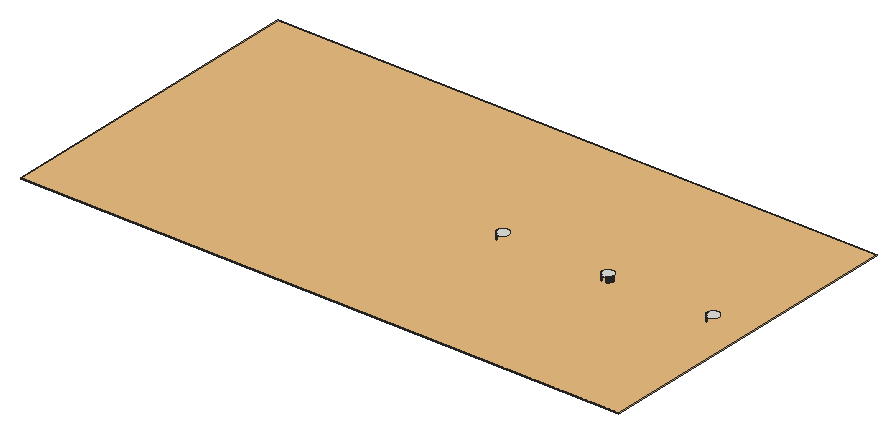
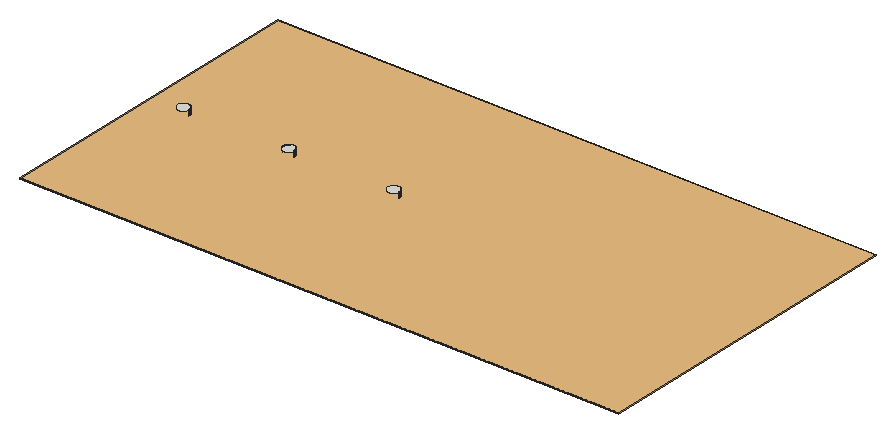
# SketchUp Ruby script. Lengths in inches.
U = 1.inch
M = Sketchup.active_model
def pt(a) = Geom::Point3d.new(a.map { |v| v * U })
def face(e, loops, mat)
  f = e.add_face(loops[0].map { |a| pt(a) })
  loops[1..].each { |l| e.add_face(l.map { |a| pt(a) }).erase! }
  f.material = f.back_material = mat if mat
  f
end
# faces: each face lists its corners as indices into pts; further lists are holes
def faces(e, pts, list, mat = nil) = list.each { |f| face(e, (f[0].is_a?(Array) ? f : [f]).map { |l| l.map { |i| pts[i] } }, mat) }
# xy, xz, yz: faces in a plane at the given z, y or x. An outline is a flat list of corners, or four numbers for a rectangle; further outlines are holes
def ring(l) = l.size == 4 ? [[l[0], l[1]], [l[2], l[1]], [l[2], l[3]], [l[0], l[3]]] : l.each_slice(2).to_a
def flat(e, list, mat, &to3) = list.each { |f| face(e, (f[0].is_a?(Array) ? f : [f]).map { |l| ring(l).map { |u, v| to3.(u, v) } }, mat) }
def xy(e, z, list, mat = nil) = flat(e, list, mat) { |x, y| [x, y, z] }
def xz(e, y, list, mat = nil) = flat(e, list, mat) { |x, z| [x, y, z] }
def yz(e, x, list, mat = nil) = flat(e, list, mat) { |y, z| [x, y, z] }
def lines(e, pts, list) = list.each { |a, b| e.add_line(pt(pts[a]), pt(pts[b])) }
# prism: a flat outline (further loops are holes) pulled along v
def prism(e, loops, v, mat = nil)
  f = face(e, loops, mat); d = Geom::Vector3d.new(v.map { |x| x * U })
  f.pushpull(f.normal.samedirection?(d) ? d.length : -d.length)
end
def box(e, o, s, mat = nil) = prism(e, [[o, [o[0] + s[0], o[1], o[2]], [o[0] + s[0], o[1] + s[1], o[2]], [o[0], o[1] + s[1], o[2]]]], [0, 0, s[2]], mat)
def at(x, y, z, deg = 0) = Geom::Transformation.translation(pt([x, y, z])) * Geom::Transformation.rotation(ORIGIN, Z_AXIS, deg.degrees)
def axes(o, x, y, z) = Geom::Transformation.new([*x, 0, *y, 0, *z, 0, *pt(o).to_a, 1])
def part(name) = M.definitions.add(name)
# library, detail: a bought-in or finely detailed component or shape, given as its bounding box
def library(name, o, s) = part(name).tap { |d| box(d.entities, o, s) }
def detail(e, o, s) = box(e.add_group.entities, o, s)
def put(e, d, t, mat = nil) = e.add_instance(d, t).tap { |i| i.material = mat if mat }
def group(e, t, mat = nil) = e.add_group.tap { |g| g.transformation = t; g.material = mat if mat }.entities
root = M.entities
M.materials.add("False Ceiling light").color = [253, 223, 143]
c1 = library("Group\#25",[0,0,-0.5],[312,168,0.5])
xy(root,234,[[214.28,251,214.2,251.01,214.12,251.01,213.96,251.03,213.89,251.04,213.73,251.08,213.66,251.09,213.58,251.11,213.5,251.14,213.43,251.16,213.36,251.1875,213.28,251.22,213.14,251.28,213.07,251.3125,213,251.35,212.93,251.39,212.86,251.42,212.79,251.47,212.73,251.51,212.66,251.55,212.36,251.8,212.19,251.97,211.99,252.21,211.95,252.27,211.9,252.34,211.86,252.4,211.74,252.61,211.71,252.68,211.67,252.75,211.61,252.89,211.58,252.97,211.56,253.04,211.53,253.12,211.51,253.19,211.49,253.27,211.47,253.34,211.46,253.42,211.44,253.5,211.43,253.58,211.42,253.65,211.41,253.73,211.41,253.81,211.4,253.89,211.4,254.125,211.41,254.2,211.41,254.28,211.42,254.36,211.43,254.4375,211.44,254.51,211.48,254.67,211.49,254.74,211.51,254.82,211.54,254.9,211.5625,254.97,211.59,255.04,211.62,255.12,211.71,255.33,211.79,255.47,211.82,255.54,211.87,255.61,211.91,255.67,211.95,255.74,212.2,256.04,212.26,256.1,212.3125,256.15,212.37,256.21,212.61,256.41,212.67,256.45,212.74,256.5,212.8,256.54,212.87,256.58,212.9375,256.62,213.01,256.66,213.08,256.69,213.15,256.73,213.29,256.79,213.37,256.82,213.44,256.84,213.52,256.87,213.59,256.89,213.67,256.91,213.74,256.93,213.82,256.94,213.9,256.96,213.98,256.97,214.05,256.98,214.13,256.99,214.21,256.99,214.29,257,214.52,257,214.6,256.99,214.68,256.99,214.84,256.97,214.91,256.96,215.07,256.92,215.14,256.91,215.22,256.89,215.3,256.86,215.37,256.84,215.44,256.8125,215.52,256.78,215.66,256.72,215.73,256.6875,215.8,256.65,215.87,256.61,215.9375,256.58,216.01,256.53,216.07,256.49,216.14,256.45,216.44,256.2,216.61,256.03,216.81,255.79,216.85,255.73,216.9,255.66,216.94,255.6,217.06,255.39,217.09,255.32,217.16,255.18,217.1875,255.11,217.22,255.03,217.24,254.96,217.27,254.88,217.29,254.81,217.31,254.73,217.33,254.66,217.34,254.58,217.36,254.5,217.37,254.42,217.38,254.35,217.39,254.27,217.39,254.19,217.4,254.11,217.4,253.875,217.39,253.8,217.39,253.72,217.38,253.64,217.37,253.5625,217.36,253.49,217.32,253.33,217.31,253.26,217.29,253.18,217.26,253.1,217.24,253.03,217.21,252.96,217.18,252.88,217.09,252.67,217.01,252.53,216.98,252.46,216.93,252.39,216.89,252.33,216.85,252.26,216.6,251.96,216.43,251.79,216.375,251.74,216.25,251.64,216.19,251.59,216.125,251.55,216.0625,251.5,216,251.46,215.79,251.34,215.72,251.31,215.65,251.27,215.51,251.21,215.43,251.18,215.36,251.16,215.28,251.13,215.21,251.11,215.13,251.09,215.06,251.07,214.98,251.06,214.9,251.04,214.82,251.03,214.75,251.02,214.67,251.01,214.59,251.01,214.51,251],[269.08,251,269,251.01,268.92,251.01,268.76,251.03,268.6875,251.04,268.61,251.06,268.53,251.08,268.46,251.09,268.38,251.11,268.3,251.14,268.23,251.16,268.16,251.1875,268.08,251.22,268.01,251.25,267.9375,251.28,267.87,251.3125,267.8,251.35,267.73,251.39,267.66,251.42,267.59,251.47,267.53,251.51,267.46,251.55,267.16,251.8,266.99,251.97,266.79,252.21,266.75,252.27,266.7,252.34,266.66,252.4,266.54,252.61,266.51,252.68,266.47,252.75,266.41,252.89,266.38,252.97,266.36,253.04,266.33,253.12,266.3125,253.19,266.29,253.27,266.27,253.34,266.26,253.42,266.24,253.5,266.23,253.58,266.22,253.65,266.21,253.73,266.21,253.81,266.2,253.89,266.2,254.125,266.21,254.2,266.21,254.28,266.22,254.36,266.23,254.4375,266.24,254.51,266.28,254.67,266.29,254.74,266.3125,254.82,266.34,254.9,266.36,254.97,266.39,255.04,266.42,255.12,266.51,255.33,266.59,255.47,266.625,255.54,266.67,255.61,266.71,255.67,266.75,255.74,267,256.04,267.17,256.21,267.41,256.41,267.47,256.45,267.54,256.5,267.6,256.54,267.81,256.66,267.88,256.69,267.95,256.73,268.09,256.79,268.17,256.82,268.24,256.84,268.32,256.87,268.39,256.89,268.47,256.91,268.54,256.93,268.62,256.94,268.7,256.96,268.78,256.97,268.85,256.98,268.93,256.99,269.01,256.99,269.09,257,269.32,257,269.4,256.99,269.48,256.99,269.64,256.97,269.71,256.96,269.87,256.92,269.94,256.91,270.02,256.89,270.1,256.86,270.17,256.84,270.24,256.8125,270.32,256.78,270.46,256.72,270.53,256.6875,270.6,256.65,270.67,256.61,270.74,256.58,270.81,256.53,270.87,256.49,270.9375,256.45,271.0625,256.35,271.12,256.3,271.24,256.2,271.41,256.03,271.61,255.79,271.65,255.73,271.7,255.66,271.74,255.6,271.86,255.39,271.89,255.32,271.93,255.25,271.99,255.11,272.02,255.03,272.04,254.96,272.07,254.88,272.09,254.81,272.11,254.73,272.13,254.66,272.14,254.58,272.16,254.5,272.17,254.42,272.18,254.35,272.1875,254.27,272.19,254.19,272.2,254.11,272.2,253.875,272.19,253.8,272.1875,253.72,272.18,253.64,272.17,253.5625,272.16,253.49,272.14,253.41,272.125,253.33,272.11,253.26,272.09,253.18,272.0625,253.1,272.04,253.03,272.01,252.96,271.98,252.88,271.89,252.67,271.81,252.53,271.78,252.46,271.73,252.39,271.69,252.33,271.65,252.26,271.4,251.96,271.23,251.79,270.99,251.59,270.93,251.55,270.86,251.5,270.8,251.46,270.59,251.34,270.52,251.31,270.45,251.27,270.31,251.21,270.23,251.18,270.16,251.16,270.08,251.13,270.01,251.11,269.93,251.09,269.86,251.07,269.78,251.06,269.7,251.04,269.55,251.02,269.47,251.01,269.39,251.01,269.3125,251],[323.875,251,323.8,251.01,323.72,251.01,323.64,251.02,323.5625,251.03,323.49,251.04,323.33,251.08,323.26,251.09,323.18,251.11,323.1,251.14,323.03,251.16,322.96,251.1875,322.88,251.22,322.74,251.28,322.67,251.3125,322.6,251.35,322.53,251.39,322.46,251.42,322.39,251.47,322.33,251.51,322.26,251.55,321.96,251.8,321.79,251.97,321.59,252.21,321.55,252.27,321.5,252.34,321.46,252.4,321.34,252.61,321.31,252.68,321.27,252.75,321.21,252.89,321.18,252.97,321.16,253.04,321.13,253.12,321.11,253.19,321.09,253.27,321.07,253.34,321.06,253.42,321.04,253.5,321.03,253.58,321.02,253.65,321.01,253.73,321.01,253.81,321,253.89,321,254.125,321.01,254.2,321.01,254.28,321.02,254.36,321.03,254.4375,321.04,254.51,321.08,254.67,321.09,254.74,321.11,254.82,321.14,254.9,321.16,254.97,321.1875,255.04,321.22,255.12,321.28,255.26,321.3125,255.33,321.35,255.4,321.39,255.47,321.42,255.54,321.47,255.61,321.51,255.67,321.55,255.74,321.8,256.04,321.97,256.21,322.21,256.41,322.27,256.45,322.34,256.5,322.4,256.54,322.61,256.66,322.68,256.69,322.75,256.73,322.89,256.79,322.97,256.82,323.04,256.84,323.12,256.87,323.19,256.89,323.27,256.91,323.34,256.93,323.42,256.94,323.5,256.96,323.58,256.97,323.65,256.98,323.73,256.99,323.81,256.99,323.89,257,324.125,257,324.2,256.99,324.28,256.99,324.36,256.98,324.4375,256.97,324.51,256.96,324.67,256.92,324.74,256.91,324.82,256.89,324.9,256.86,324.97,256.84,325.04,256.8125,325.12,256.78,325.26,256.72,325.33,256.6875,325.4,256.65,325.47,256.61,325.54,256.58,325.61,256.53,325.67,256.49,325.74,256.45,326.04,256.2,326.21,256.03,326.41,255.79,326.45,255.73,326.5,255.66,326.54,255.6,326.66,255.39,326.69,255.32,326.73,255.25,326.79,255.11,326.82,255.03,326.84,254.96,326.87,254.88,326.89,254.81,326.91,254.73,326.93,254.66,326.94,254.58,326.96,254.5,326.97,254.42,326.98,254.35,326.99,254.27,326.99,254.19,327,254.11,327,253.875,326.99,253.8,326.99,253.72,326.98,253.64,326.97,253.5625,326.96,253.49,326.92,253.33,326.91,253.26,326.89,253.18,326.86,253.1,326.84,253.03,326.8125,252.96,326.78,252.88,326.72,252.74,326.6875,252.67,326.65,252.6,326.61,252.53,326.58,252.46,326.53,252.39,326.49,252.33,326.45,252.26,326.2,251.96,326.03,251.79,325.79,251.59,325.73,251.55,325.66,251.5,325.6,251.46,325.39,251.34,325.32,251.31,325.25,251.27,325.11,251.21,325.03,251.18,324.96,251.16,324.88,251.13,324.81,251.11,324.73,251.09,324.66,251.07,324.58,251.06,324.5,251.04,324.42,251.03,324.35,251.02,324.27,251.01,324.19,251.01,324.11,251]])
yz(root,211.4,[[253.89,231,253.97,234],[253.97,231,254.05,234],[254.05,231,254.125,234]])
yz(root,211.41,[[253.73,231,253.81,234],[254.2,231,254.28,234]])
yz(root,266.2,[[253.89,231,253.97,234],[253.97,231,254.05,234],[254.05,231,254.125,234]])
yz(root,266.21,[[253.73,231,253.81,234],[254.2,231,254.28,234]])
yz(root,272.2,[[253.875,231,253.95,234],[253.95,231,254.03,234],[254.03,231,254.11,234]])
yz(root,321,[[253.89,231,253.97,234],[253.97,231,254.05,234],[254.05,231,254.125,234]])
yz(root,321.01,[[253.73,231,253.81,234],[254.2,231,254.28,234]])
p = [[268.3,251.14,231],[268.23,251.16,231],[268.23,251.16,234],[268.3,251.14,234],[213.21,251.25,231],[213.14,251.28,231],
  [213.14,251.28,234],[213.21,251.25,234],[213.28,251.22,231],[213.28,251.22,234],[213.36,251.1875,231],[213.36,251.1875,234],
  [213.43,251.16,231],[213.43,251.16,234],[268.01,251.25,231],[267.9375,251.28,231],[267.9375,251.28,234],[268.01,251.25,234],
  [268.08,251.22,231],[268.08,251.22,234],[268.16,251.1875,231],[268.16,251.1875,234],[270.23,251.18,231],[270.16,251.16,231],
  [270.16,251.16,234],[270.23,251.18,234],[270.31,251.21,231],[270.31,251.21,234],[270.38,251.24,231],[270.38,251.24,234],
  [270.45,251.27,231],[270.45,251.27,234],[322.81,251.25,231],[322.74,251.28,231],[322.74,251.28,234],[322.81,251.25,234],
  [322.88,251.22,231],[322.88,251.22,234],[322.96,251.1875,231],[322.96,251.1875,234],[323.03,251.16,231],[323.03,251.16,234],
  [213,251.35,231],[212.93,251.39,231],[212.93,251.39,234],[213,251.35,234],[213.07,251.3125,231],[213.07,251.3125,234],
  [267.8,251.35,231],[267.73,251.39,231],[267.73,251.39,234],[267.8,251.35,234],[267.87,251.3125,231],[267.87,251.3125,234],
  [270.52,251.31,231],[270.52,251.31,234],[270.59,251.34,231],[270.59,251.34,234],[270.66,251.38,231],[270.66,251.38,234],
  [322.6,251.35,231],[322.53,251.39,231],[322.53,251.39,234],[322.6,251.35,234],[322.67,251.3125,231],[322.67,251.3125,234],
  [212.86,251.42,231],[212.79,251.47,231],[212.79,251.47,234],[212.86,251.42,234],[267.66,251.42,231],[267.59,251.47,231],
  [267.59,251.47,234],[267.66,251.42,234],[270.73,251.42,231],[270.73,251.42,234],[270.8,251.46,231],[270.8,251.46,234],
  [322.46,251.42,231],[322.39,251.47,231],[322.39,251.47,234],[322.46,251.42,234],[212.73,251.51,231],[212.73,251.51,234],
  [212.66,251.55,231],[212.66,251.55,234],[267.53,251.51,231],[267.53,251.51,234],[267.46,251.55,231],[267.46,251.55,234],
  [270.86,251.5,231],[270.86,251.5,234],[270.93,251.55,231],[270.93,251.55,234],[270.99,251.59,231],[270.99,251.59,234],
  [322.33,251.51,231],[322.33,251.51,234],[322.26,251.55,231],[322.26,251.55,234],[212.6,251.6,231],[212.54,251.65,231],
  [212.54,251.65,234],[212.6,251.6,234],[212.48,251.7,231],[212.48,251.7,234],[267.4,251.6,231],[267.34,251.65,231],
  [267.34,251.65,234],[267.4,251.6,234],[267.28,251.7,231],[267.28,251.7,234],[271.05,251.64,231],[271.05,251.64,234],
  [271.11,251.69,231],[271.11,251.69,234],[322.2,251.6,231],[322.14,251.65,231],[322.14,251.65,234],[322.2,251.6,234],
  [322.08,251.7,231],[322.08,251.7,234],[212.42,251.75,231],[212.42,251.75,234],[212.36,251.8,231],[212.36,251.8,234],
  [267.22,251.75,231],[267.22,251.75,234],[267.16,251.8,231],[267.16,251.8,234],[271.17,251.74,231],[271.17,251.74,234],
  [271.23,251.79,231],[271.23,251.79,234],[322.02,251.75,231],[322.02,251.75,234],[321.96,251.8,231],[321.96,251.8,234],
  [212.3,251.86,231],[212.3,251.86,234],[267.1,251.86,231],[267.1,251.86,234],[271.29,251.85,231],[271.29,251.85,234],
  [271.34,251.9,231],[271.34,251.9,234],[321.9,251.86,231],[321.9,251.86,234],[212.25,251.91,231],[212.25,251.91,234],
  [212.19,251.97,231],[212.19,251.97,234],[267.05,251.91,231],[267.05,251.91,234],[266.99,251.97,231],[266.99,251.97,234],
  [271.4,251.96,231],[271.4,251.96,234],[321.85,251.91,231],[321.85,251.91,234],[321.79,251.97,231],[321.79,251.97,234],
  [212.14,252.03,231],[212.14,252.03,234],[212.09,252.09,231],[212.09,252.09,234],[266.94,252.03,231],[266.94,252.03,234],
  [266.89,252.09,231],[266.89,252.09,234],[271.45,252.02,231],[271.45,252.02,234],[271.5,252.08,231],[271.5,252.08,234],
  [321.74,252.03,231],[321.74,252.03,234],[321.69,252.09,231],[321.69,252.09,234],[212.04,252.15,231],[212.04,252.15,234],
  [211.99,252.21,231],[211.99,252.21,234],[266.84,252.15,231],[266.84,252.15,234],[266.79,252.21,231],[266.79,252.21,234],
  [271.55,252.14,231],[271.55,252.14,234],[271.6,252.2,231],[271.6,252.2,234],[321.64,252.15,231],[321.64,252.15,234],
  [321.59,252.21,231],[321.59,252.21,234],[211.95,252.27,231],[211.95,252.27,234],[266.75,252.27,231],[266.75,252.27,234],
  [271.65,252.26,231],[271.65,252.26,234],[321.55,252.27,231],[321.55,252.27,234],[211.9,252.34,231],[211.9,252.34,234],
  [211.86,252.4,231],[211.86,252.4,234],[266.7,252.34,231],[266.7,252.34,234],[266.66,252.4,231],[266.66,252.4,234],
  [271.69,252.33,231],[271.69,252.33,234],[271.73,252.39,231],[271.73,252.39,234],[321.5,252.34,231],[321.5,252.34,234],
  [321.46,252.4,231],[321.46,252.4,234],[211.82,252.47,231],[211.82,252.47,234],[266.62,252.47,231],[266.62,252.47,234],
  [271.78,252.46,231],[271.78,252.46,234],[321.42,252.47,231],[321.42,252.47,234],[211.78,252.54,231],[211.74,252.61,231],
  [211.74,252.61,234],[211.78,252.54,234],[266.58,252.54,231],[266.54,252.61,231],[266.54,252.61,234],[266.58,252.54,234],
  [271.81,252.53,231],[271.81,252.53,234],[271.85,252.6,231],[271.85,252.6,234],[321.38,252.54,231],[321.34,252.61,231],
  [321.34,252.61,234],[321.38,252.54,234],[211.71,252.68,231],[211.71,252.68,234],[266.51,252.68,231],[266.51,252.68,234],
  [271.89,252.67,231],[271.89,252.67,234],[321.31,252.68,231],[321.31,252.68,234],[211.67,252.75,231],[211.64,252.82,231],
  [211.64,252.82,234],[211.67,252.75,234],[266.47,252.75,231],[266.44,252.82,231],[266.44,252.82,234],[266.47,252.75,234],
  [271.92,252.74,231],[271.92,252.74,234],[271.95,252.81,231],[271.95,252.81,234],[321.27,252.75,231],[321.24,252.82,231],
  [321.24,252.82,234],[321.27,252.75,234],[211.61,252.89,231],[211.61,252.89,234],[266.41,252.89,231],[266.41,252.89,234],
  [271.98,252.88,231],[271.98,252.88,234],[321.21,252.89,231],[321.21,252.89,234],[211.58,252.97,231],[211.58,252.97,234],
  [266.38,252.97,231],[266.38,252.97,234],[272.01,252.96,231],[272.01,252.96,234],[321.18,252.97,231],[321.18,252.97,234],
  [211.56,253.04,231],[211.53,253.12,231],[211.53,253.12,234],[211.56,253.04,234],[266.36,253.04,231],[266.33,253.12,231],
  [266.33,253.12,234],[266.36,253.04,234],[272.04,253.03,231],[272.04,253.03,234],[272.0625,253.1,231],[272.0625,253.1,234],
  [321.16,253.04,231],[321.13,253.12,231],[321.13,253.12,234],[321.16,253.04,234],[211.51,253.19,231],[211.51,253.19,234],
  [266.3125,253.19,231],[266.3125,253.19,234],[272.09,253.18,231],[272.09,253.18,234],[321.11,253.19,231],[321.11,253.19,234],
  [211.49,253.27,231],[211.49,253.27,234],[266.29,253.27,231],[266.29,253.27,234],[272.11,253.26,231],[272.11,253.26,234],
  [321.09,253.27,231],[321.09,253.27,234],[211.47,253.34,231],[211.47,253.34,234],[211.46,253.42,231],[211.46,253.42,234],
  [266.27,253.34,231],[266.27,253.34,234],[266.26,253.42,231],[266.26,253.42,234],[272.125,253.33,231],[272.125,253.33,234],
  [272.14,253.41,231],[272.14,253.41,234],[321.07,253.34,231],[321.07,253.34,234],[321.06,253.42,231],[321.06,253.42,234],
  [211.44,253.5,231],[211.44,253.5,234],[266.24,253.5,231],[266.24,253.5,234],[272.16,253.49,231],[272.16,253.49,234],
  [321.04,253.5,231],[321.04,253.5,234],[211.43,253.58,231],[211.43,253.58,234],[266.23,253.58,231],[266.23,253.58,234],
  [272.17,253.5625,231],[272.17,253.5625,234],[321.03,253.58,231],[321.03,253.58,234],[211.42,253.65,231],[211.42,253.65,234],
  [266.22,253.65,231],[266.22,253.65,234],[272.18,253.64,231],[272.18,253.64,234],[272.1875,253.72,231],[272.1875,253.72,234],
  [321.02,253.65,231],[321.02,253.65,234],[211.41,253.73,231],[211.41,253.73,234],[266.21,253.73,231],[266.21,253.73,234],
  [272.19,253.8,231],[272.19,253.8,234],[321.01,253.73,231],[321.01,253.73,234],[211.41,253.81,231],[211.4,253.89,231],
  [211.4,253.89,234],[211.41,253.81,234],[266.21,253.81,231],[266.2,253.89,231],[266.2,253.89,234],[266.21,253.81,234],
  [272.2,253.875,231],[272.2,253.875,234],[321.01,253.81,231],[321,253.89,231],[321,253.89,234],[321.01,253.81,234],
  [211.4,254.125,231],[211.41,254.2,231],[211.41,254.2,234],[211.4,254.125,234],[266.2,254.125,231],[266.21,254.2,231],
  [266.21,254.2,234],[266.2,254.125,234],[272.19,254.19,231],[272.2,254.11,231],[272.2,254.11,234],[272.19,254.19,234],
  [321,254.125,231],[321.01,254.2,231],[321.01,254.2,234],[321,254.125,234],[272.1875,254.27,231],[272.1875,254.27,234],
  [211.41,254.28,231],[211.42,254.36,231],[211.42,254.36,234],[211.41,254.28,234],[266.21,254.28,231],[266.22,254.36,231],
  [266.22,254.36,234],[266.21,254.28,234],[272.18,254.35,231],[272.18,254.35,234],[272.17,254.42,231],[272.17,254.42,234],
  [321.01,254.28,231],[321.02,254.36,231],[321.02,254.36,234],[321.01,254.28,234],[211.43,254.4375,231],[211.43,254.4375,234]]
faces(root,p,[[0,1,2,3],[4,5,6,7],[8,4,7,9],[10,8,9,11],[12,10,11,13],[14,15,16,17],[18,14,17,19],[20,18,19,21],
  [1,20,21,2],[22,23,24,25],[26,22,25,27],[28,26,27,29],[30,28,29,31],[32,33,34,35],[36,32,35,37],[38,36,37,39],
  [40,38,39,41],[42,43,44,45],[46,42,45,47],[5,46,47,6],[48,49,50,51],[52,48,51,53],[15,52,53,16],[54,30,31,55],
  [56,54,55,57],[58,56,57,59],[60,61,62,63],[64,60,63,65],[33,64,65,34],[66,67,68,69],[43,66,69,44],[70,71,72,73],
  [49,70,73,50],[74,58,59,75],[76,74,75,77],[78,79,80,81],[61,78,81,62],[67,82,83,68],[82,84,85,83],[71,86,87,72],
  [86,88,89,87],[90,76,77,91],[92,90,91,93],[94,92,93,95],[79,96,97,80],[96,98,99,97],[100,101,102,103],[101,104,105,102],
  [84,100,103,85],[106,107,108,109],[107,110,111,108],[88,106,109,89],[112,94,95,113],[114,112,113,115],[116,117,118,119],[117,120,121,118],
  [98,116,119,99],[104,122,123,105],[122,124,125,123],[110,126,127,111],[126,128,129,127],[130,114,115,131],[132,130,131,133],[120,134,135,121],
  [134,136,137,135],[124,138,139,125],[128,140,141,129],[142,132,133,143],[144,142,143,145],[136,146,147,137],[138,148,149,139],[148,150,151,149],
  [140,152,153,141],[152,154,155,153],[156,144,145,157],[146,158,159,147],[158,160,161,159],[150,162,163,151],[162,164,165,163],[154,166,167,155],
  [166,168,169,167],[170,156,157,171],[172,170,171,173],[160,174,175,161],[174,176,177,175],[164,178,179,165],[178,180,181,179],[168,182,183,169],
  [182,184,185,183],[186,172,173,187],[188,186,187,189],[176,190,191,177],[190,192,193,191],[180,194,195,181],[184,196,197,185],[198,188,189,199],
  [192,200,201,193],[194,202,203,195],[202,204,205,203],[196,206,207,197],[206,208,209,207],[210,198,199,211],[212,210,211,213],[200,214,215,201],
  [214,216,217,215],[204,218,219,205],[208,220,221,209],[222,212,213,223],[216,224,225,217],[226,227,228,229],[218,226,229,219],[230,231,232,233],
  [220,230,233,221],[234,222,223,235],[236,234,235,237],[238,239,240,241],[224,238,241,225],[227,242,243,228],[231,244,245,232],[246,236,237,247],
  [239,248,249,240],[250,251,252,253],[242,250,253,243],[254,255,256,257],[244,254,257,245],[258,246,247,259],[260,258,259,261],[262,263,264,265],
  [248,262,265,249],[251,266,267,252],[255,268,269,256],[270,260,261,271],[263,272,273,264],[266,274,275,267],[268,276,277,269],[278,270,271,279],
  [272,280,281,273],[282,283,284,285],[274,282,285,275],[286,287,288,289],[276,286,289,277],[290,278,279,291],[292,290,291,293],[294,295,296,297],
  [280,294,297,281],[283,298,299,284],[287,300,301,288],[302,292,293,303],[295,304,305,296],[298,306,307,299],[300,308,309,301],[310,302,303,311],
  [304,312,313,305],[306,314,315,307],[314,316,317,315],[308,318,319,309],[318,320,321,319],[322,310,311,323],[324,322,323,325],[312,326,327,313],
  [326,328,329,327],[316,330,331,317],[320,332,333,321],[334,324,325,335],[328,336,337,329],[330,338,339,331],[332,340,341,333],[342,334,335,343],
  [336,344,345,337],[338,346,347,339],[340,348,349,341],[350,342,343,351],[352,350,351,353],[344,354,355,345],[346,356,357,347],[348,358,359,349],
  [360,352,353,361],[354,362,363,355],[364,365,366,367],[368,369,370,371],[372,360,361,373],[374,375,376,377],[378,379,380,381],[382,383,384,385],
  [386,387,388,389],[390,391,392,393],[394,386,389,395],[396,397,398,399],[400,401,402,403],[404,394,395,405],[406,404,405,407],[408,409,410,411],
  [397,412,413,398]])
put(root,c1,at(30,170,231.5),"False Ceiling light")
